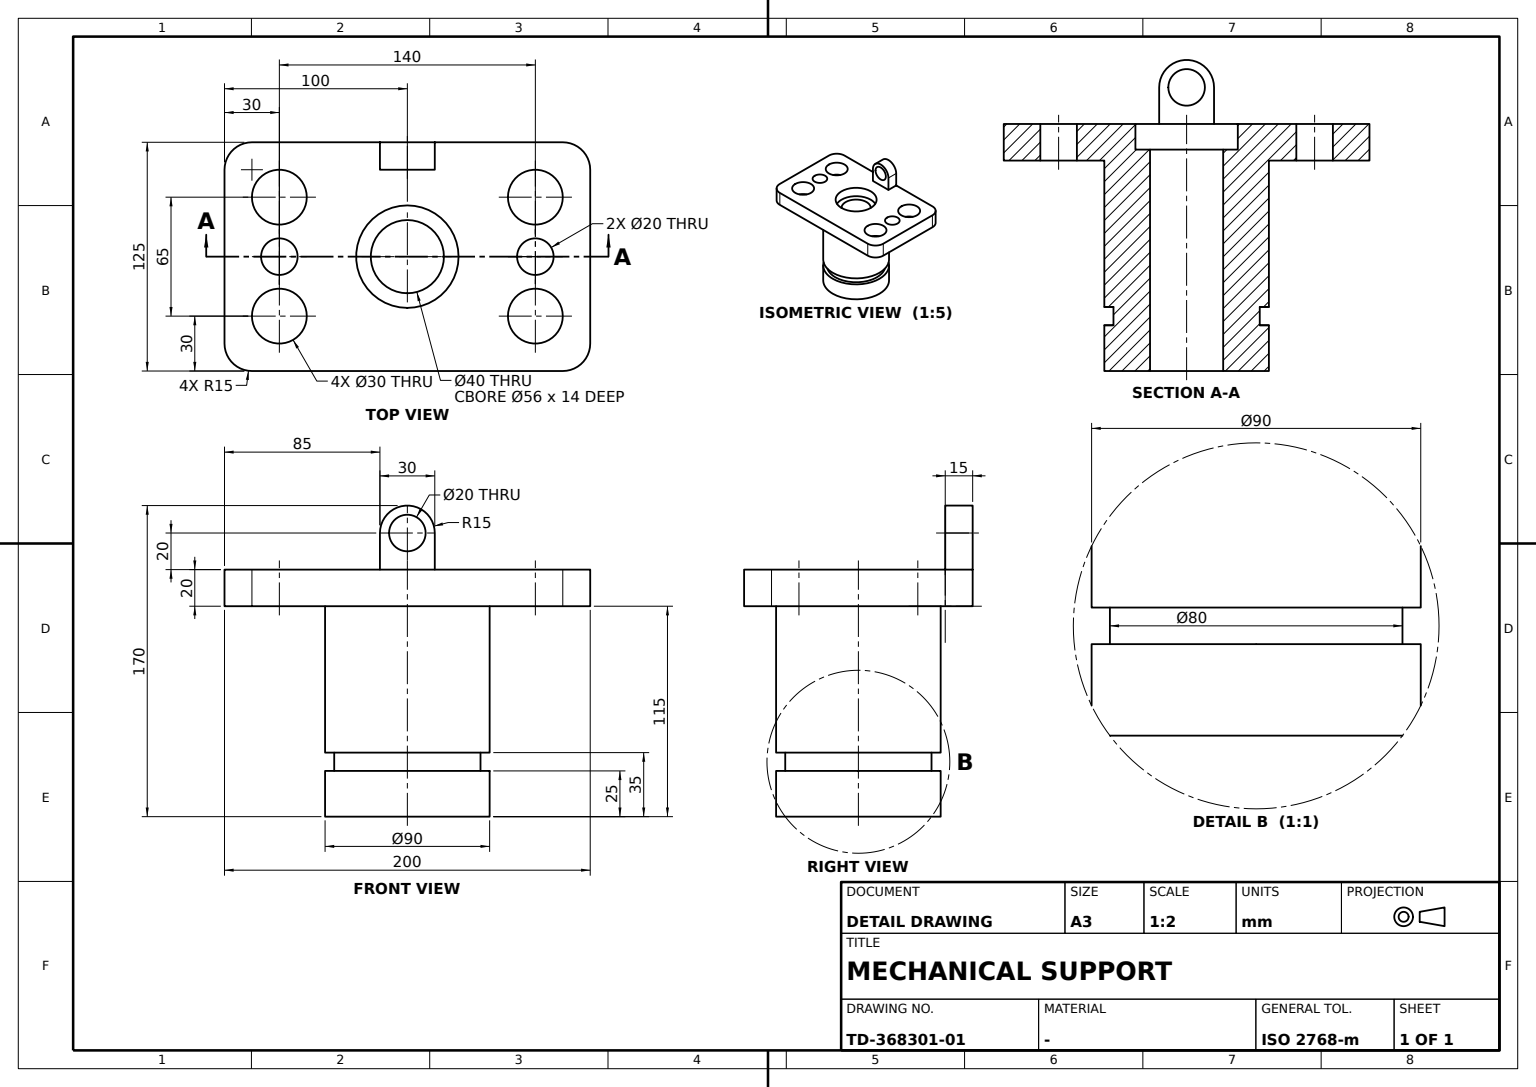
ISO-10303-21;
HEADER;
FILE_DESCRIPTION((''),'2;1');
FILE_NAME('','',(''),(''),'','','');
FILE_SCHEMA(('AUTOMOTIVE_DESIGN'));
ENDSEC;
DATA;
#1=APPLICATION_CONTEXT('');
#2=PRODUCT_CONTEXT('',#1,'mechanical');
#3=PRODUCT('','','',(#2));
#4=PRODUCT_DEFINITION_FORMATION('','',#3);
#5=PRODUCT_DEFINITION_CONTEXT('',#1,'design');
#6=PRODUCT_DEFINITION('','',#4,#5);
#7=PRODUCT_DEFINITION_SHAPE('','',#6);
#8=(LENGTH_UNIT()NAMED_UNIT(*)SI_UNIT(.MILLI.,.METRE.));
#9=(NAMED_UNIT(*)PLANE_ANGLE_UNIT()SI_UNIT($,.RADIAN.));
#10=(NAMED_UNIT(*)SI_UNIT($,.STERADIAN.)SOLID_ANGLE_UNIT());
#11=UNCERTAINTY_MEASURE_WITH_UNIT(LENGTH_MEASURE(1.E-05),#8,'distance_accuracy_value','');
#12=(GEOMETRIC_REPRESENTATION_CONTEXT(3)GLOBAL_UNCERTAINTY_ASSIGNED_CONTEXT((#11))GLOBAL_UNIT_ASSIGNED_CONTEXT((#8,#9,#10))REPRESENTATION_CONTEXT('',''));
#13=CARTESIAN_POINT('',(85.,-62.5,135.));
#14=VERTEX_POINT('',#13);
#15=CARTESIAN_POINT('',(85.,-62.5,115.));
#16=VERTEX_POINT('',#15);
#17=CARTESIAN_POINT('',(85.,-62.5,125.));
#18=DIRECTION('',(0.,0.,-1.));
#19=VECTOR('',#18,1000.);
#20=LINE('',#17,#19);
#21=EDGE_CURVE('',#14,#16,#20,.T.);
#22=ORIENTED_EDGE('',*,*,#21,.F.);
#23=CARTESIAN_POINT('',(-85.,-62.5,135.));
#24=VERTEX_POINT('',#23);
#25=CARTESIAN_POINT('',(0.,-62.5,135.));
#26=DIRECTION('',(1.,0.,0.));
#27=VECTOR('',#26,1000.);
#28=LINE('',#25,#27);
#29=EDGE_CURVE('',#24,#14,#28,.T.);
#30=ORIENTED_EDGE('',*,*,#29,.F.);
#31=CARTESIAN_POINT('',(-85.,-62.5,115.));
#32=VERTEX_POINT('',#31);
#33=CARTESIAN_POINT('',(-85.,-62.5,125.));
#34=LINE('',#33,#19);
#35=EDGE_CURVE('',#24,#32,#34,.T.);
#36=ORIENTED_EDGE('',*,*,#35,.T.);
#37=CARTESIAN_POINT('',(0.,-62.5,115.));
#38=LINE('',#37,#27);
#39=EDGE_CURVE('',#32,#16,#38,.T.);
#40=ORIENTED_EDGE('',*,*,#39,.T.);
#41=EDGE_LOOP('',(#22,#30,#36,#40));
#42=FACE_OUTER_BOUND('',#41,.T.);
#43=DIRECTION('',(0.,-1.,0.));
#44=DIRECTION('',(-1.,0.,0.));
#45=AXIS2_PLACEMENT_3D('',#13,#43,#44);
#46=PLANE('',#45);
#47=ADVANCED_FACE('',(#42),#46,.T.);
#48=CARTESIAN_POINT('',(55.,32.5,135.));
#49=VERTEX_POINT('',#48);
#50=CARTESIAN_POINT('',(85.,32.5,135.));
#51=VERTEX_POINT('',#50);
#52=CARTESIAN_POINT('',(70.,32.5,135.));
#53=DIRECTION('',(0.,0.,1.));
#54=AXIS2_PLACEMENT_3D('',#52,#53,#26);
#55=CIRCLE('',#54,15.);
#56=EDGE_CURVE('',#49,#51,#55,.T.);
#57=ORIENTED_EDGE('',*,*,#56,.F.);
#58=EDGE_CURVE('',#51,#49,#55,.T.);
#59=ORIENTED_EDGE('',*,*,#58,.F.);
#60=EDGE_LOOP('',(#57,#59));
#61=FACE_BOUND('',#60,.T.);
#62=CARTESIAN_POINT('',(0.,28.,135.));
#63=VERTEX_POINT('',#62);
#64=CARTESIAN_POINT('',(0.,-28.,135.));
#65=VERTEX_POINT('',#64);
#66=CARTESIAN_POINT('',(0.,0.,135.));
#67=AXIS2_PLACEMENT_3D('',#66,#53,#26);
#68=CIRCLE('',#67,28.);
#69=EDGE_CURVE('',#63,#65,#68,.T.);
#70=ORIENTED_EDGE('',*,*,#69,.F.);
#71=CARTESIAN_POINT('',(28.,0.,135.));
#72=VERTEX_POINT('',#71);
#73=EDGE_CURVE('',#72,#63,#68,.T.);
#74=ORIENTED_EDGE('',*,*,#73,.F.);
#75=EDGE_CURVE('',#65,#72,#68,.T.);
#76=ORIENTED_EDGE('',*,*,#75,.F.);
#77=EDGE_LOOP('',(#70,#74,#76));
#78=FACE_BOUND('',#77,.T.);
#79=CARTESIAN_POINT('',(-85.,-32.5,135.));
#80=VERTEX_POINT('',#79);
#81=CARTESIAN_POINT('',(-55.,-32.5,135.));
#82=VERTEX_POINT('',#81);
#83=CARTESIAN_POINT('',(-70.,-32.5,135.));
#84=AXIS2_PLACEMENT_3D('',#83,#53,#26);
#85=CIRCLE('',#84,15.);
#86=EDGE_CURVE('',#80,#82,#85,.T.);
#87=ORIENTED_EDGE('',*,*,#86,.F.);
#88=EDGE_CURVE('',#82,#80,#85,.T.);
#89=ORIENTED_EDGE('',*,*,#88,.F.);
#90=EDGE_LOOP('',(#87,#89));
#91=FACE_BOUND('',#90,.T.);
#92=CARTESIAN_POINT('',(-55.,32.5,135.));
#93=VERTEX_POINT('',#92);
#94=CARTESIAN_POINT('',(-85.,32.5,135.));
#95=VERTEX_POINT('',#94);
#96=CARTESIAN_POINT('',(-70.,32.5,135.));
#97=AXIS2_PLACEMENT_3D('',#96,#53,#26);
#98=CIRCLE('',#97,15.);
#99=EDGE_CURVE('',#93,#95,#98,.T.);
#100=ORIENTED_EDGE('',*,*,#99,.F.);
#101=EDGE_CURVE('',#95,#93,#98,.T.);
#102=ORIENTED_EDGE('',*,*,#101,.F.);
#103=EDGE_LOOP('',(#100,#102));
#104=FACE_BOUND('',#103,.T.);
#105=CARTESIAN_POINT('',(-80.,0.,135.));
#106=VERTEX_POINT('',#105);
#107=CARTESIAN_POINT('',(-60.,0.,135.));
#108=VERTEX_POINT('',#107);
#109=CARTESIAN_POINT('',(-70.,0.,135.));
#110=AXIS2_PLACEMENT_3D('',#109,#53,#26);
#111=CIRCLE('',#110,10.);
#112=EDGE_CURVE('',#106,#108,#111,.T.);
#113=ORIENTED_EDGE('',*,*,#112,.F.);
#114=EDGE_CURVE('',#108,#106,#111,.T.);
#115=ORIENTED_EDGE('',*,*,#114,.F.);
#116=EDGE_LOOP('',(#113,#115));
#117=FACE_BOUND('',#116,.T.);
#118=CARTESIAN_POINT('',(55.,-32.5,135.));
#119=VERTEX_POINT('',#118);
#120=CARTESIAN_POINT('',(85.,-32.5,135.));
#121=VERTEX_POINT('',#120);
#122=CARTESIAN_POINT('',(70.,-32.5,135.));
#123=AXIS2_PLACEMENT_3D('',#122,#53,#26);
#124=CIRCLE('',#123,15.);
#125=EDGE_CURVE('',#119,#121,#124,.T.);
#126=ORIENTED_EDGE('',*,*,#125,.F.);
#127=EDGE_CURVE('',#121,#119,#124,.T.);
#128=ORIENTED_EDGE('',*,*,#127,.F.);
#129=EDGE_LOOP('',(#126,#128));
#130=FACE_BOUND('',#129,.T.);
#131=CARTESIAN_POINT('',(80.,0.,135.));
#132=VERTEX_POINT('',#131);
#133=CARTESIAN_POINT('',(60.,0.,135.));
#134=VERTEX_POINT('',#133);
#135=CARTESIAN_POINT('',(70.,0.,135.));
#136=AXIS2_PLACEMENT_3D('',#135,#53,#26);
#137=CIRCLE('',#136,10.);
#138=EDGE_CURVE('',#132,#134,#137,.T.);
#139=ORIENTED_EDGE('',*,*,#138,.F.);
#140=EDGE_CURVE('',#134,#132,#137,.T.);
#141=ORIENTED_EDGE('',*,*,#140,.F.);
#142=EDGE_LOOP('',(#139,#141));
#143=FACE_BOUND('',#142,.T.);
#144=CARTESIAN_POINT('',(-100.,-47.5,135.));
#145=VERTEX_POINT('',#144);
#146=CARTESIAN_POINT('',(-85.,-47.5,135.));
#147=AXIS2_PLACEMENT_3D('',#146,#53,#26);
#148=CIRCLE('',#147,15.);
#149=EDGE_CURVE('',#145,#24,#148,.T.);
#150=ORIENTED_EDGE('',*,*,#149,.T.);
#151=ORIENTED_EDGE('',*,*,#29,.T.);
#152=CARTESIAN_POINT('',(100.,-47.5,135.));
#153=VERTEX_POINT('',#152);
#154=CARTESIAN_POINT('',(85.,-47.5,135.));
#155=AXIS2_PLACEMENT_3D('',#154,#53,#26);
#156=CIRCLE('',#155,15.);
#157=EDGE_CURVE('',#14,#153,#156,.T.);
#158=ORIENTED_EDGE('',*,*,#157,.T.);
#159=CARTESIAN_POINT('',(100.,47.5,135.));
#160=VERTEX_POINT('',#159);
#161=CARTESIAN_POINT('',(100.,0.,135.));
#162=DIRECTION('',(0.,1.,0.));
#163=VECTOR('',#162,1000.);
#164=LINE('',#161,#163);
#165=EDGE_CURVE('',#153,#160,#164,.T.);
#166=ORIENTED_EDGE('',*,*,#165,.T.);
#167=CARTESIAN_POINT('',(85.,62.5,135.));
#168=VERTEX_POINT('',#167);
#169=CARTESIAN_POINT('',(85.,47.5,135.));
#170=AXIS2_PLACEMENT_3D('',#169,#53,#26);
#171=CIRCLE('',#170,15.);
#172=EDGE_CURVE('',#160,#168,#171,.T.);
#173=ORIENTED_EDGE('',*,*,#172,.T.);
#174=CARTESIAN_POINT('',(15.,62.5,135.));
#175=VERTEX_POINT('',#174);
#176=CARTESIAN_POINT('',(50.,62.5,135.));
#177=VECTOR('',#44,1000.);
#178=LINE('',#176,#177);
#179=EDGE_CURVE('',#168,#175,#178,.T.);
#180=ORIENTED_EDGE('',*,*,#179,.T.);
#181=CARTESIAN_POINT('',(15.,47.5,135.));
#182=VERTEX_POINT('',#181);
#183=CARTESIAN_POINT('',(15.,55.,135.));
#184=VECTOR('',#43,1000.);
#185=LINE('',#183,#184);
#186=EDGE_CURVE('',#175,#182,#185,.T.);
#187=ORIENTED_EDGE('',*,*,#186,.T.);
#188=CARTESIAN_POINT('',(-15.,47.5,135.));
#189=VERTEX_POINT('',#188);
#190=CARTESIAN_POINT('',(0.,47.5,135.));
#191=LINE('',#190,#177);
#192=EDGE_CURVE('',#182,#189,#191,.T.);
#193=ORIENTED_EDGE('',*,*,#192,.T.);
#194=CARTESIAN_POINT('',(-15.,62.5,135.));
#195=VERTEX_POINT('',#194);
#196=CARTESIAN_POINT('',(-15.,55.,135.));
#197=LINE('',#196,#184);
#198=EDGE_CURVE('',#195,#189,#197,.T.);
#199=ORIENTED_EDGE('',*,*,#198,.F.);
#200=CARTESIAN_POINT('',(-85.,62.5,135.));
#201=VERTEX_POINT('',#200);
#202=CARTESIAN_POINT('',(-50.,62.5,135.));
#203=LINE('',#202,#177);
#204=EDGE_CURVE('',#195,#201,#203,.T.);
#205=ORIENTED_EDGE('',*,*,#204,.T.);
#206=CARTESIAN_POINT('',(-100.,47.5,135.));
#207=VERTEX_POINT('',#206);
#208=CARTESIAN_POINT('',(-85.,47.5,135.));
#209=AXIS2_PLACEMENT_3D('',#208,#53,#26);
#210=CIRCLE('',#209,15.);
#211=EDGE_CURVE('',#201,#207,#210,.T.);
#212=ORIENTED_EDGE('',*,*,#211,.T.);
#213=CARTESIAN_POINT('',(-100.,0.,135.));
#214=LINE('',#213,#184);
#215=EDGE_CURVE('',#207,#145,#214,.T.);
#216=ORIENTED_EDGE('',*,*,#215,.T.);
#217=EDGE_LOOP('',(#150,#151,#158,#166,#173,#180,#187,#193,#199,#205,#212,#216));
#218=FACE_OUTER_BOUND('',#217,.T.);
#219=AXIS2_PLACEMENT_3D('',#62,#53,#26);
#220=PLANE('',#219);
#221=ADVANCED_FACE('',(#61,#78,#91,#104,#117,#130,#143,#218),#220,.T.);
#222=CARTESIAN_POINT('',(0.,-40.,25.));
#223=VERTEX_POINT('',#222);
#224=CARTESIAN_POINT('',(40.,0.,25.));
#225=VERTEX_POINT('',#224);
#226=CARTESIAN_POINT('',(0.,0.,25.));
#227=AXIS2_PLACEMENT_3D('',#226,#53,#26);
#228=CIRCLE('',#227,40.);
#229=EDGE_CURVE('',#223,#225,#228,.T.);
#230=ORIENTED_EDGE('',*,*,#229,.F.);
#231=CARTESIAN_POINT('',(0.,40.,25.));
#232=VERTEX_POINT('',#231);
#233=EDGE_CURVE('',#232,#223,#228,.T.);
#234=ORIENTED_EDGE('',*,*,#233,.F.);
#235=EDGE_CURVE('',#225,#232,#228,.T.);
#236=ORIENTED_EDGE('',*,*,#235,.F.);
#237=EDGE_LOOP('',(#230,#234,#236));
#238=FACE_BOUND('',#237,.T.);
#239=CARTESIAN_POINT('',(0.,-45.,25.));
#240=VERTEX_POINT('',#239);
#241=CARTESIAN_POINT('',(45.,0.,25.));
#242=VERTEX_POINT('',#241);
#243=CIRCLE('',#227,45.);
#244=EDGE_CURVE('',#240,#242,#243,.T.);
#245=ORIENTED_EDGE('',*,*,#244,.T.);
#246=CARTESIAN_POINT('',(0.,45.,25.));
#247=VERTEX_POINT('',#246);
#248=EDGE_CURVE('',#242,#247,#243,.T.);
#249=ORIENTED_EDGE('',*,*,#248,.T.);
#250=EDGE_CURVE('',#247,#240,#243,.T.);
#251=ORIENTED_EDGE('',*,*,#250,.T.);
#252=EDGE_LOOP('',(#245,#249,#251));
#253=FACE_OUTER_BOUND('',#252,.T.);
#254=AXIS2_PLACEMENT_3D('',#231,#53,#26);
#255=PLANE('',#254);
#256=ADVANCED_FACE('',(#238,#253),#255,.T.);
#257=CARTESIAN_POINT('',(-85.,62.5,115.));
#258=VERTEX_POINT('',#257);
#259=CARTESIAN_POINT('',(-100.,47.5,115.));
#260=VERTEX_POINT('',#259);
#261=CARTESIAN_POINT('',(-85.,47.5,115.));
#262=AXIS2_PLACEMENT_3D('',#261,#53,#26);
#263=CIRCLE('',#262,15.);
#264=EDGE_CURVE('',#258,#260,#263,.T.);
#265=ORIENTED_EDGE('',*,*,#264,.T.);
#266=CARTESIAN_POINT('',(-100.,47.5,125.));
#267=LINE('',#266,#19);
#268=EDGE_CURVE('',#207,#260,#267,.T.);
#269=ORIENTED_EDGE('',*,*,#268,.F.);
#270=ORIENTED_EDGE('',*,*,#211,.F.);
#271=CARTESIAN_POINT('',(-85.,62.5,125.));
#272=LINE('',#271,#19);
#273=EDGE_CURVE('',#201,#258,#272,.T.);
#274=ORIENTED_EDGE('',*,*,#273,.T.);
#275=EDGE_LOOP('',(#265,#269,#270,#274));
#276=FACE_OUTER_BOUND('',#275,.T.);
#277=CARTESIAN_POINT('',(-85.,47.5,125.));
#278=AXIS2_PLACEMENT_3D('',#277,#18,#26);
#279=CYLINDRICAL_SURFACE('',#278,15.);
#280=ADVANCED_FACE('',(#276),#279,.T.);
#281=CARTESIAN_POINT('',(45.,0.,115.));
#282=VERTEX_POINT('',#281);
#283=CARTESIAN_POINT('',(0.,45.,115.));
#284=VERTEX_POINT('',#283);
#285=CARTESIAN_POINT('',(0.,0.,115.));
#286=AXIS2_PLACEMENT_3D('',#285,#53,#26);
#287=CIRCLE('',#286,45.);
#288=EDGE_CURVE('',#282,#284,#287,.T.);
#289=ORIENTED_EDGE('',*,*,#288,.F.);
#290=CARTESIAN_POINT('',(45.,0.,35.));
#291=VERTEX_POINT('',#290);
#292=CARTESIAN_POINT('',(45.,0.,67.5));
#293=LINE('',#292,#19);
#294=EDGE_CURVE('',#282,#291,#293,.T.);
#295=ORIENTED_EDGE('',*,*,#294,.T.);
#296=CARTESIAN_POINT('',(0.,45.,35.));
#297=VERTEX_POINT('',#296);
#298=CARTESIAN_POINT('',(0.,0.,35.));
#299=AXIS2_PLACEMENT_3D('',#298,#53,#26);
#300=CIRCLE('',#299,45.);
#301=EDGE_CURVE('',#291,#297,#300,.T.);
#302=ORIENTED_EDGE('',*,*,#301,.T.);
#303=CARTESIAN_POINT('',(0.,45.,67.5));
#304=VECTOR('',#53,1000.);
#305=LINE('',#303,#304);
#306=EDGE_CURVE('',#297,#284,#305,.T.);
#307=ORIENTED_EDGE('',*,*,#306,.T.);
#308=EDGE_LOOP('',(#289,#295,#302,#307));
#309=FACE_OUTER_BOUND('',#308,.T.);
#310=CARTESIAN_POINT('',(0.,0.,67.5));
#311=AXIS2_PLACEMENT_3D('',#310,#18,#26);
#312=CYLINDRICAL_SURFACE('',#311,45.);
#313=ADVANCED_FACE('',(#309),#312,.T.);
#314=CARTESIAN_POINT('',(80.,0.,115.));
#315=VERTEX_POINT('',#314);
#316=CARTESIAN_POINT('',(60.,0.,115.));
#317=VERTEX_POINT('',#316);
#318=CARTESIAN_POINT('',(70.,0.,115.));
#319=AXIS2_PLACEMENT_3D('',#318,#53,#26);
#320=CIRCLE('',#319,10.);
#321=EDGE_CURVE('',#315,#317,#320,.T.);
#322=ORIENTED_EDGE('',*,*,#321,.F.);
#323=CARTESIAN_POINT('',(80.,0.,125.));
#324=LINE('',#323,#19);
#325=EDGE_CURVE('',#132,#315,#324,.T.);
#326=ORIENTED_EDGE('',*,*,#325,.F.);
#327=ORIENTED_EDGE('',*,*,#138,.T.);
#328=CARTESIAN_POINT('',(60.,0.,125.));
#329=LINE('',#328,#19);
#330=EDGE_CURVE('',#134,#317,#329,.T.);
#331=ORIENTED_EDGE('',*,*,#330,.T.);
#332=EDGE_LOOP('',(#322,#326,#327,#331));
#333=FACE_OUTER_BOUND('',#332,.T.);
#334=CARTESIAN_POINT('',(70.,0.,125.));
#335=AXIS2_PLACEMENT_3D('',#334,#18,#26);
#336=CYLINDRICAL_SURFACE('',#335,10.);
#337=ADVANCED_FACE('',(#333),#336,.F.);
#338=CARTESIAN_POINT('',(85.,-32.5,115.));
#339=VERTEX_POINT('',#338);
#340=CARTESIAN_POINT('',(85.,-32.5,125.));
#341=LINE('',#340,#19);
#342=EDGE_CURVE('',#121,#339,#341,.T.);
#343=ORIENTED_EDGE('',*,*,#342,.T.);
#344=CARTESIAN_POINT('',(55.,-32.5,115.));
#345=VERTEX_POINT('',#344);
#346=CARTESIAN_POINT('',(70.,-32.5,115.));
#347=AXIS2_PLACEMENT_3D('',#346,#53,#26);
#348=CIRCLE('',#347,15.);
#349=EDGE_CURVE('',#345,#339,#348,.T.);
#350=ORIENTED_EDGE('',*,*,#349,.F.);
#351=CARTESIAN_POINT('',(55.,-32.5,125.));
#352=LINE('',#351,#19);
#353=EDGE_CURVE('',#119,#345,#352,.T.);
#354=ORIENTED_EDGE('',*,*,#353,.F.);
#355=ORIENTED_EDGE('',*,*,#125,.T.);
#356=EDGE_LOOP('',(#343,#350,#354,#355));
#357=FACE_OUTER_BOUND('',#356,.T.);
#358=CARTESIAN_POINT('',(70.,-32.5,125.));
#359=AXIS2_PLACEMENT_3D('',#358,#18,#26);
#360=CYLINDRICAL_SURFACE('',#359,15.);
#361=ADVANCED_FACE('',(#357),#360,.F.);
#362=CARTESIAN_POINT('',(40.,0.,35.));
#363=VERTEX_POINT('',#362);
#364=CARTESIAN_POINT('',(40.,0.,67.5));
#365=LINE('',#364,#19);
#366=EDGE_CURVE('',#363,#225,#365,.T.);
#367=ORIENTED_EDGE('',*,*,#366,.F.);
#368=CARTESIAN_POINT('',(0.,-40.,35.));
#369=VERTEX_POINT('',#368);
#370=CIRCLE('',#299,40.);
#371=EDGE_CURVE('',#369,#363,#370,.T.);
#372=ORIENTED_EDGE('',*,*,#371,.F.);
#373=CARTESIAN_POINT('',(0.,-40.,30.));
#374=LINE('',#373,#304);
#375=EDGE_CURVE('',#223,#369,#374,.T.);
#376=ORIENTED_EDGE('',*,*,#375,.F.);
#377=ORIENTED_EDGE('',*,*,#229,.T.);
#378=EDGE_LOOP('',(#367,#372,#376,#377));
#379=FACE_OUTER_BOUND('',#378,.T.);
#380=CYLINDRICAL_SURFACE('',#311,40.);
#381=ADVANCED_FACE('',(#379),#380,.T.);
#382=CARTESIAN_POINT('',(-10.,47.5,155.));
#383=VERTEX_POINT('',#382);
#384=CARTESIAN_POINT('',(10.,47.5,155.));
#385=VERTEX_POINT('',#384);
#386=CARTESIAN_POINT('',(0.,47.5,155.));
#387=AXIS2_PLACEMENT_3D('',#386,#162,#44);
#388=CIRCLE('',#387,10.);
#389=EDGE_CURVE('',#383,#385,#388,.T.);
#390=ORIENTED_EDGE('',*,*,#389,.T.);
#391=EDGE_CURVE('',#385,#383,#388,.T.);
#392=ORIENTED_EDGE('',*,*,#391,.T.);
#393=EDGE_LOOP('',(#390,#392));
#394=FACE_BOUND('',#393,.T.);
#395=CARTESIAN_POINT('',(15.,47.5,155.));
#396=VERTEX_POINT('',#395);
#397=CARTESIAN_POINT('',(15.,47.5,145.));
#398=LINE('',#397,#19);
#399=EDGE_CURVE('',#396,#182,#398,.T.);
#400=ORIENTED_EDGE('',*,*,#399,.F.);
#401=CARTESIAN_POINT('',(-15.,47.5,155.));
#402=VERTEX_POINT('',#401);
#403=CIRCLE('',#387,15.);
#404=EDGE_CURVE('',#402,#396,#403,.T.);
#405=ORIENTED_EDGE('',*,*,#404,.F.);
#406=CARTESIAN_POINT('',(-15.,47.5,145.));
#407=LINE('',#406,#304);
#408=EDGE_CURVE('',#189,#402,#407,.T.);
#409=ORIENTED_EDGE('',*,*,#408,.F.);
#410=ORIENTED_EDGE('',*,*,#192,.F.);
#411=EDGE_LOOP('',(#400,#405,#409,#410));
#412=FACE_OUTER_BOUND('',#411,.T.);
#413=CARTESIAN_POINT('',(0.,47.5,0.));
#414=AXIS2_PLACEMENT_3D('',#413,#162,#44);
#415=PLANE('',#414);
#416=ADVANCED_FACE('',(#394,#412),#415,.F.);
#417=ORIENTED_EDGE('',*,*,#21,.T.);
#418=CARTESIAN_POINT('',(100.,-47.5,115.));
#419=VERTEX_POINT('',#418);
#420=CARTESIAN_POINT('',(85.,-47.5,115.));
#421=AXIS2_PLACEMENT_3D('',#420,#53,#26);
#422=CIRCLE('',#421,15.);
#423=EDGE_CURVE('',#16,#419,#422,.T.);
#424=ORIENTED_EDGE('',*,*,#423,.T.);
#425=CARTESIAN_POINT('',(100.,-47.5,125.));
#426=LINE('',#425,#19);
#427=EDGE_CURVE('',#153,#419,#426,.T.);
#428=ORIENTED_EDGE('',*,*,#427,.F.);
#429=ORIENTED_EDGE('',*,*,#157,.F.);
#430=EDGE_LOOP('',(#417,#424,#428,#429));
#431=FACE_OUTER_BOUND('',#430,.T.);
#432=CARTESIAN_POINT('',(85.,-47.5,125.));
#433=AXIS2_PLACEMENT_3D('',#432,#18,#26);
#434=CYLINDRICAL_SURFACE('',#433,15.);
#435=ADVANCED_FACE('',(#431),#434,.T.);
#436=ORIENTED_EDGE('',*,*,#114,.T.);
#437=CARTESIAN_POINT('',(-80.,0.,115.));
#438=VERTEX_POINT('',#437);
#439=CARTESIAN_POINT('',(-80.,0.,125.));
#440=LINE('',#439,#19);
#441=EDGE_CURVE('',#106,#438,#440,.T.);
#442=ORIENTED_EDGE('',*,*,#441,.T.);
#443=CARTESIAN_POINT('',(-60.,0.,115.));
#444=VERTEX_POINT('',#443);
#445=CARTESIAN_POINT('',(-70.,0.,115.));
#446=AXIS2_PLACEMENT_3D('',#445,#53,#26);
#447=CIRCLE('',#446,10.);
#448=EDGE_CURVE('',#444,#438,#447,.T.);
#449=ORIENTED_EDGE('',*,*,#448,.F.);
#450=CARTESIAN_POINT('',(-60.,0.,125.));
#451=LINE('',#450,#19);
#452=EDGE_CURVE('',#108,#444,#451,.T.);
#453=ORIENTED_EDGE('',*,*,#452,.F.);
#454=EDGE_LOOP('',(#436,#442,#449,#453));
#455=FACE_OUTER_BOUND('',#454,.T.);
#456=CARTESIAN_POINT('',(-70.,0.,125.));
#457=AXIS2_PLACEMENT_3D('',#456,#18,#26);
#458=CYLINDRICAL_SURFACE('',#457,10.);
#459=ADVANCED_FACE('',(#455),#458,.F.);
#460=ORIENTED_EDGE('',*,*,#56,.T.);
#461=CARTESIAN_POINT('',(85.,32.5,115.));
#462=VERTEX_POINT('',#461);
#463=CARTESIAN_POINT('',(85.,32.5,125.));
#464=LINE('',#463,#19);
#465=EDGE_CURVE('',#51,#462,#464,.T.);
#466=ORIENTED_EDGE('',*,*,#465,.T.);
#467=CARTESIAN_POINT('',(55.,32.5,115.));
#468=VERTEX_POINT('',#467);
#469=CARTESIAN_POINT('',(70.,32.5,115.));
#470=AXIS2_PLACEMENT_3D('',#469,#53,#26);
#471=CIRCLE('',#470,15.);
#472=EDGE_CURVE('',#468,#462,#471,.T.);
#473=ORIENTED_EDGE('',*,*,#472,.F.);
#474=CARTESIAN_POINT('',(55.,32.5,125.));
#475=LINE('',#474,#19);
#476=EDGE_CURVE('',#49,#468,#475,.T.);
#477=ORIENTED_EDGE('',*,*,#476,.F.);
#478=EDGE_LOOP('',(#460,#466,#473,#477));
#479=FACE_OUTER_BOUND('',#478,.T.);
#480=CARTESIAN_POINT('',(70.,32.5,125.));
#481=AXIS2_PLACEMENT_3D('',#480,#18,#26);
#482=CYLINDRICAL_SURFACE('',#481,15.);
#483=ADVANCED_FACE('',(#479),#482,.F.);
#484=ORIENTED_EDGE('',*,*,#404,.T.);
#485=CARTESIAN_POINT('',(15.,62.5,155.));
#486=VERTEX_POINT('',#485);
#487=CARTESIAN_POINT('',(15.,55.,155.));
#488=LINE('',#487,#184);
#489=EDGE_CURVE('',#486,#396,#488,.T.);
#490=ORIENTED_EDGE('',*,*,#489,.F.);
#491=CARTESIAN_POINT('',(-15.,62.5,155.));
#492=VERTEX_POINT('',#491);
#493=CARTESIAN_POINT('',(0.,62.5,155.));
#494=AXIS2_PLACEMENT_3D('',#493,#162,#44);
#495=CIRCLE('',#494,15.);
#496=EDGE_CURVE('',#492,#486,#495,.T.);
#497=ORIENTED_EDGE('',*,*,#496,.F.);
#498=CARTESIAN_POINT('',(-15.,55.,155.));
#499=LINE('',#498,#184);
#500=EDGE_CURVE('',#492,#402,#499,.T.);
#501=ORIENTED_EDGE('',*,*,#500,.T.);
#502=EDGE_LOOP('',(#484,#490,#497,#501));
#503=FACE_OUTER_BOUND('',#502,.T.);
#504=CARTESIAN_POINT('',(0.,55.,155.));
#505=AXIS2_PLACEMENT_3D('',#504,#43,#44);
#506=CYLINDRICAL_SURFACE('',#505,15.);
#507=ADVANCED_FACE('',(#503),#506,.T.);
#508=CARTESIAN_POINT('',(0.,20.,121.));
#509=VERTEX_POINT('',#508);
#510=CARTESIAN_POINT('',(0.,20.,0.));
#511=VERTEX_POINT('',#510);
#512=CARTESIAN_POINT('',(0.,20.,60.5));
#513=LINE('',#512,#19);
#514=EDGE_CURVE('',#509,#511,#513,.T.);
#515=ORIENTED_EDGE('',*,*,#514,.T.);
#516=CARTESIAN_POINT('',(20.,0.,0.));
#517=VERTEX_POINT('',#516);
#518=CARTESIAN_POINT('',(0.,0.,0.));
#519=AXIS2_PLACEMENT_3D('',#518,#53,#26);
#520=CIRCLE('',#519,20.);
#521=EDGE_CURVE('',#517,#511,#520,.T.);
#522=ORIENTED_EDGE('',*,*,#521,.F.);
#523=CARTESIAN_POINT('',(20.,0.,121.));
#524=VERTEX_POINT('',#523);
#525=CARTESIAN_POINT('',(20.,0.,67.5));
#526=LINE('',#525,#19);
#527=EDGE_CURVE('',#524,#517,#526,.T.);
#528=ORIENTED_EDGE('',*,*,#527,.F.);
#529=CARTESIAN_POINT('',(0.,0.,121.));
#530=AXIS2_PLACEMENT_3D('',#529,#53,#26);
#531=CIRCLE('',#530,20.);
#532=EDGE_CURVE('',#524,#509,#531,.T.);
#533=ORIENTED_EDGE('',*,*,#532,.T.);
#534=EDGE_LOOP('',(#515,#522,#528,#533));
#535=FACE_OUTER_BOUND('',#534,.T.);
#536=CYLINDRICAL_SURFACE('',#311,20.);
#537=ADVANCED_FACE('',(#535),#536,.F.);
#538=ORIENTED_EDGE('',*,*,#325,.T.);
#539=EDGE_CURVE('',#317,#315,#320,.T.);
#540=ORIENTED_EDGE('',*,*,#539,.F.);
#541=ORIENTED_EDGE('',*,*,#330,.F.);
#542=ORIENTED_EDGE('',*,*,#140,.T.);
#543=EDGE_LOOP('',(#538,#540,#541,#542));
#544=FACE_OUTER_BOUND('',#543,.T.);
#545=ADVANCED_FACE('',(#544),#336,.F.);
#546=CARTESIAN_POINT('',(85.,62.5,115.));
#547=VERTEX_POINT('',#546);
#548=CARTESIAN_POINT('',(85.,62.5,125.));
#549=LINE('',#548,#19);
#550=EDGE_CURVE('',#168,#547,#549,.T.);
#551=ORIENTED_EDGE('',*,*,#550,.F.);
#552=ORIENTED_EDGE('',*,*,#172,.F.);
#553=CARTESIAN_POINT('',(100.,47.5,115.));
#554=VERTEX_POINT('',#553);
#555=CARTESIAN_POINT('',(100.,47.5,125.));
#556=LINE('',#555,#19);
#557=EDGE_CURVE('',#160,#554,#556,.T.);
#558=ORIENTED_EDGE('',*,*,#557,.T.);
#559=CARTESIAN_POINT('',(85.,47.5,115.));
#560=AXIS2_PLACEMENT_3D('',#559,#53,#26);
#561=CIRCLE('',#560,15.);
#562=EDGE_CURVE('',#554,#547,#561,.T.);
#563=ORIENTED_EDGE('',*,*,#562,.T.);
#564=EDGE_LOOP('',(#551,#552,#558,#563));
#565=FACE_OUTER_BOUND('',#564,.T.);
#566=CARTESIAN_POINT('',(85.,47.5,125.));
#567=AXIS2_PLACEMENT_3D('',#566,#18,#26);
#568=CYLINDRICAL_SURFACE('',#567,15.);
#569=ADVANCED_FACE('',(#565),#568,.T.);
#570=ORIENTED_EDGE('',*,*,#375,.T.);
#571=CARTESIAN_POINT('',(0.,40.,35.));
#572=VERTEX_POINT('',#571);
#573=EDGE_CURVE('',#572,#369,#370,.T.);
#574=ORIENTED_EDGE('',*,*,#573,.F.);
#575=CARTESIAN_POINT('',(0.,40.,30.));
#576=LINE('',#575,#304);
#577=EDGE_CURVE('',#232,#572,#576,.T.);
#578=ORIENTED_EDGE('',*,*,#577,.F.);
#579=ORIENTED_EDGE('',*,*,#233,.T.);
#580=EDGE_LOOP('',(#570,#574,#578,#579));
#581=FACE_OUTER_BOUND('',#580,.T.);
#582=ADVANCED_FACE('',(#581),#380,.T.);
#583=CARTESIAN_POINT('',(28.,0.,121.));
#584=VERTEX_POINT('',#583);
#585=CARTESIAN_POINT('',(0.,28.,121.));
#586=VERTEX_POINT('',#585);
#587=CIRCLE('',#530,28.);
#588=EDGE_CURVE('',#584,#586,#587,.T.);
#589=ORIENTED_EDGE('',*,*,#588,.F.);
#590=CARTESIAN_POINT('',(28.,0.,67.5));
#591=LINE('',#590,#19);
#592=EDGE_CURVE('',#72,#584,#591,.T.);
#593=ORIENTED_EDGE('',*,*,#592,.F.);
#594=ORIENTED_EDGE('',*,*,#73,.T.);
#595=CARTESIAN_POINT('',(0.,28.,128.));
#596=LINE('',#595,#19);
#597=EDGE_CURVE('',#63,#586,#596,.T.);
#598=ORIENTED_EDGE('',*,*,#597,.T.);
#599=EDGE_LOOP('',(#589,#593,#594,#598));
#600=FACE_OUTER_BOUND('',#599,.T.);
#601=CYLINDRICAL_SURFACE('',#311,28.);
#602=ADVANCED_FACE('',(#600),#601,.F.);
#603=ORIENTED_EDGE('',*,*,#288,.T.);
#604=CARTESIAN_POINT('',(0.,-45.,115.));
#605=VERTEX_POINT('',#604);
#606=EDGE_CURVE('',#284,#605,#287,.T.);
#607=ORIENTED_EDGE('',*,*,#606,.T.);
#608=EDGE_CURVE('',#605,#282,#287,.T.);
#609=ORIENTED_EDGE('',*,*,#608,.T.);
#610=EDGE_LOOP('',(#603,#607,#609));
#611=FACE_BOUND('',#610,.T.);
#612=CARTESIAN_POINT('',(-85.,-32.5,115.));
#613=VERTEX_POINT('',#612);
#614=CARTESIAN_POINT('',(-55.,-32.5,115.));
#615=VERTEX_POINT('',#614);
#616=CARTESIAN_POINT('',(-70.,-32.5,115.));
#617=AXIS2_PLACEMENT_3D('',#616,#53,#26);
#618=CIRCLE('',#617,15.);
#619=EDGE_CURVE('',#613,#615,#618,.T.);
#620=ORIENTED_EDGE('',*,*,#619,.T.);
#621=EDGE_CURVE('',#615,#613,#618,.T.);
#622=ORIENTED_EDGE('',*,*,#621,.T.);
#623=EDGE_LOOP('',(#620,#622));
#624=FACE_BOUND('',#623,.T.);
#625=EDGE_CURVE('',#462,#468,#471,.T.);
#626=ORIENTED_EDGE('',*,*,#625,.T.);
#627=ORIENTED_EDGE('',*,*,#472,.T.);
#628=EDGE_LOOP('',(#626,#627));
#629=FACE_BOUND('',#628,.T.);
#630=EDGE_CURVE('',#339,#345,#348,.T.);
#631=ORIENTED_EDGE('',*,*,#630,.T.);
#632=ORIENTED_EDGE('',*,*,#349,.T.);
#633=EDGE_LOOP('',(#631,#632));
#634=FACE_BOUND('',#633,.T.);
#635=CARTESIAN_POINT('',(0.,62.5,115.));
#636=LINE('',#635,#177);
#637=EDGE_CURVE('',#547,#258,#636,.T.);
#638=ORIENTED_EDGE('',*,*,#637,.F.);
#639=ORIENTED_EDGE('',*,*,#562,.F.);
#640=CARTESIAN_POINT('',(100.,0.,115.));
#641=LINE('',#640,#163);
#642=EDGE_CURVE('',#419,#554,#641,.T.);
#643=ORIENTED_EDGE('',*,*,#642,.F.);
#644=ORIENTED_EDGE('',*,*,#423,.F.);
#645=ORIENTED_EDGE('',*,*,#39,.F.);
#646=CARTESIAN_POINT('',(-100.,-47.5,115.));
#647=VERTEX_POINT('',#646);
#648=CARTESIAN_POINT('',(-85.,-47.5,115.));
#649=AXIS2_PLACEMENT_3D('',#648,#53,#26);
#650=CIRCLE('',#649,15.);
#651=EDGE_CURVE('',#647,#32,#650,.T.);
#652=ORIENTED_EDGE('',*,*,#651,.F.);
#653=CARTESIAN_POINT('',(-100.,0.,115.));
#654=LINE('',#653,#184);
#655=EDGE_CURVE('',#260,#647,#654,.T.);
#656=ORIENTED_EDGE('',*,*,#655,.F.);
#657=ORIENTED_EDGE('',*,*,#264,.F.);
#658=EDGE_LOOP('',(#638,#639,#643,#644,#645,#652,#656,#657));
#659=FACE_OUTER_BOUND('',#658,.T.);
#660=ORIENTED_EDGE('',*,*,#321,.T.);
#661=ORIENTED_EDGE('',*,*,#539,.T.);
#662=EDGE_LOOP('',(#660,#661));
#663=FACE_BOUND('',#662,.T.);
#664=ORIENTED_EDGE('',*,*,#448,.T.);
#665=EDGE_CURVE('',#438,#444,#447,.T.);
#666=ORIENTED_EDGE('',*,*,#665,.T.);
#667=EDGE_LOOP('',(#664,#666));
#668=FACE_BOUND('',#667,.T.);
#669=CARTESIAN_POINT('',(-55.,32.5,115.));
#670=VERTEX_POINT('',#669);
#671=CARTESIAN_POINT('',(-85.,32.5,115.));
#672=VERTEX_POINT('',#671);
#673=CARTESIAN_POINT('',(-70.,32.5,115.));
#674=AXIS2_PLACEMENT_3D('',#673,#53,#26);
#675=CIRCLE('',#674,15.);
#676=EDGE_CURVE('',#670,#672,#675,.T.);
#677=ORIENTED_EDGE('',*,*,#676,.T.);
#678=EDGE_CURVE('',#672,#670,#675,.T.);
#679=ORIENTED_EDGE('',*,*,#678,.T.);
#680=EDGE_LOOP('',(#677,#679));
#681=FACE_BOUND('',#680,.T.);
#682=PLANE('',#286);
#683=ADVANCED_FACE('',(#611,#624,#629,#634,#659,#663,#668,#681),#682,.F.);
#684=ORIENTED_EDGE('',*,*,#101,.T.);
#685=CARTESIAN_POINT('',(-55.,32.5,125.));
#686=LINE('',#685,#19);
#687=EDGE_CURVE('',#93,#670,#686,.T.);
#688=ORIENTED_EDGE('',*,*,#687,.T.);
#689=ORIENTED_EDGE('',*,*,#678,.F.);
#690=CARTESIAN_POINT('',(-85.,32.5,125.));
#691=LINE('',#690,#19);
#692=EDGE_CURVE('',#95,#672,#691,.T.);
#693=ORIENTED_EDGE('',*,*,#692,.F.);
#694=EDGE_LOOP('',(#684,#688,#689,#693));
#695=FACE_OUTER_BOUND('',#694,.T.);
#696=CARTESIAN_POINT('',(-70.,32.5,125.));
#697=AXIS2_PLACEMENT_3D('',#696,#18,#26);
#698=CYLINDRICAL_SURFACE('',#697,15.);
#699=ADVANCED_FACE('',(#695),#698,.F.);
#700=ORIENTED_EDGE('',*,*,#389,.F.);
#701=CARTESIAN_POINT('',(-10.,62.5,155.));
#702=VERTEX_POINT('',#701);
#703=CARTESIAN_POINT('',(-10.,55.,155.));
#704=LINE('',#703,#184);
#705=EDGE_CURVE('',#702,#383,#704,.T.);
#706=ORIENTED_EDGE('',*,*,#705,.F.);
#707=CARTESIAN_POINT('',(10.,62.5,155.));
#708=VERTEX_POINT('',#707);
#709=CIRCLE('',#494,10.);
#710=EDGE_CURVE('',#702,#708,#709,.T.);
#711=ORIENTED_EDGE('',*,*,#710,.T.);
#712=CARTESIAN_POINT('',(10.,55.,155.));
#713=LINE('',#712,#184);
#714=EDGE_CURVE('',#708,#385,#713,.T.);
#715=ORIENTED_EDGE('',*,*,#714,.T.);
#716=EDGE_LOOP('',(#700,#706,#711,#715));
#717=FACE_OUTER_BOUND('',#716,.T.);
#718=CYLINDRICAL_SURFACE('',#505,10.);
#719=ADVANCED_FACE('',(#717),#718,.F.);
#720=CARTESIAN_POINT('',(0.,-45.,35.));
#721=VERTEX_POINT('',#720);
#722=CARTESIAN_POINT('',(0.,-45.,67.5));
#723=LINE('',#722,#304);
#724=EDGE_CURVE('',#721,#605,#723,.T.);
#725=ORIENTED_EDGE('',*,*,#724,.F.);
#726=EDGE_CURVE('',#721,#291,#300,.T.);
#727=ORIENTED_EDGE('',*,*,#726,.T.);
#728=ORIENTED_EDGE('',*,*,#294,.F.);
#729=ORIENTED_EDGE('',*,*,#608,.F.);
#730=EDGE_LOOP('',(#725,#727,#728,#729));
#731=FACE_OUTER_BOUND('',#730,.T.);
#732=ADVANCED_FACE('',(#731),#312,.T.);
#733=ORIENTED_EDGE('',*,*,#86,.T.);
#734=CARTESIAN_POINT('',(-55.,-32.5,125.));
#735=LINE('',#734,#19);
#736=EDGE_CURVE('',#82,#615,#735,.T.);
#737=ORIENTED_EDGE('',*,*,#736,.T.);
#738=ORIENTED_EDGE('',*,*,#619,.F.);
#739=CARTESIAN_POINT('',(-85.,-32.5,125.));
#740=LINE('',#739,#19);
#741=EDGE_CURVE('',#80,#613,#740,.T.);
#742=ORIENTED_EDGE('',*,*,#741,.F.);
#743=EDGE_LOOP('',(#733,#737,#738,#742));
#744=FACE_OUTER_BOUND('',#743,.T.);
#745=CARTESIAN_POINT('',(-70.,-32.5,125.));
#746=AXIS2_PLACEMENT_3D('',#745,#18,#26);
#747=CYLINDRICAL_SURFACE('',#746,15.);
#748=ADVANCED_FACE('',(#744),#747,.F.);
#749=CARTESIAN_POINT('',(0.,-45.,0.));
#750=VERTEX_POINT('',#749);
#751=EDGE_CURVE('',#750,#240,#723,.T.);
#752=ORIENTED_EDGE('',*,*,#751,.F.);
#753=CARTESIAN_POINT('',(45.,0.,0.));
#754=VERTEX_POINT('',#753);
#755=CIRCLE('',#519,45.);
#756=EDGE_CURVE('',#750,#754,#755,.T.);
#757=ORIENTED_EDGE('',*,*,#756,.T.);
#758=EDGE_CURVE('',#242,#754,#293,.T.);
#759=ORIENTED_EDGE('',*,*,#758,.F.);
#760=ORIENTED_EDGE('',*,*,#244,.F.);
#761=EDGE_LOOP('',(#752,#757,#759,#760));
#762=FACE_OUTER_BOUND('',#761,.T.);
#763=ADVANCED_FACE('',(#762),#312,.T.);
#764=ORIENTED_EDGE('',*,*,#248,.F.);
#765=ORIENTED_EDGE('',*,*,#758,.T.);
#766=CARTESIAN_POINT('',(0.,45.,0.));
#767=VERTEX_POINT('',#766);
#768=EDGE_CURVE('',#754,#767,#755,.T.);
#769=ORIENTED_EDGE('',*,*,#768,.T.);
#770=EDGE_CURVE('',#767,#247,#305,.T.);
#771=ORIENTED_EDGE('',*,*,#770,.T.);
#772=EDGE_LOOP('',(#764,#765,#769,#771));
#773=FACE_OUTER_BOUND('',#772,.T.);
#774=ADVANCED_FACE('',(#773),#312,.T.);
#775=EDGE_CURVE('',#297,#721,#300,.T.);
#776=ORIENTED_EDGE('',*,*,#775,.T.);
#777=ORIENTED_EDGE('',*,*,#724,.T.);
#778=ORIENTED_EDGE('',*,*,#606,.F.);
#779=ORIENTED_EDGE('',*,*,#306,.F.);
#780=EDGE_LOOP('',(#776,#777,#778,#779));
#781=FACE_OUTER_BOUND('',#780,.T.);
#782=ADVANCED_FACE('',(#781),#312,.T.);
#783=ORIENTED_EDGE('',*,*,#705,.T.);
#784=ORIENTED_EDGE('',*,*,#391,.F.);
#785=ORIENTED_EDGE('',*,*,#714,.F.);
#786=EDGE_CURVE('',#708,#702,#709,.T.);
#787=ORIENTED_EDGE('',*,*,#786,.T.);
#788=EDGE_LOOP('',(#783,#784,#785,#787));
#789=FACE_OUTER_BOUND('',#788,.T.);
#790=ADVANCED_FACE('',(#789),#718,.F.);
#791=ORIENTED_EDGE('',*,*,#399,.T.);
#792=ORIENTED_EDGE('',*,*,#186,.F.);
#793=CARTESIAN_POINT('',(15.,62.5,145.));
#794=LINE('',#793,#19);
#795=EDGE_CURVE('',#486,#175,#794,.T.);
#796=ORIENTED_EDGE('',*,*,#795,.F.);
#797=ORIENTED_EDGE('',*,*,#489,.T.);
#798=EDGE_LOOP('',(#791,#792,#796,#797));
#799=FACE_OUTER_BOUND('',#798,.T.);
#800=AXIS2_PLACEMENT_3D('',#174,#26,#53);
#801=PLANE('',#800);
#802=ADVANCED_FACE('',(#799),#801,.T.);
#803=ORIENTED_EDGE('',*,*,#366,.T.);
#804=ORIENTED_EDGE('',*,*,#235,.T.);
#805=ORIENTED_EDGE('',*,*,#577,.T.);
#806=EDGE_CURVE('',#363,#572,#370,.T.);
#807=ORIENTED_EDGE('',*,*,#806,.F.);
#808=EDGE_LOOP('',(#803,#804,#805,#807));
#809=FACE_OUTER_BOUND('',#808,.T.);
#810=ADVANCED_FACE('',(#809),#380,.T.);
#811=ORIENTED_EDGE('',*,*,#655,.T.);
#812=CARTESIAN_POINT('',(-100.,-47.5,125.));
#813=LINE('',#812,#19);
#814=EDGE_CURVE('',#145,#647,#813,.T.);
#815=ORIENTED_EDGE('',*,*,#814,.F.);
#816=ORIENTED_EDGE('',*,*,#215,.F.);
#817=ORIENTED_EDGE('',*,*,#268,.T.);
#818=EDGE_LOOP('',(#811,#815,#816,#817));
#819=FACE_OUTER_BOUND('',#818,.T.);
#820=AXIS2_PLACEMENT_3D('',#144,#44,#162);
#821=PLANE('',#820);
#822=ADVANCED_FACE('',(#819),#821,.T.);
#823=ORIENTED_EDGE('',*,*,#665,.F.);
#824=ORIENTED_EDGE('',*,*,#441,.F.);
#825=ORIENTED_EDGE('',*,*,#112,.T.);
#826=ORIENTED_EDGE('',*,*,#452,.T.);
#827=EDGE_LOOP('',(#823,#824,#825,#826));
#828=FACE_OUTER_BOUND('',#827,.T.);
#829=ADVANCED_FACE('',(#828),#458,.F.);
#830=ORIENTED_EDGE('',*,*,#768,.F.);
#831=ORIENTED_EDGE('',*,*,#756,.F.);
#832=EDGE_CURVE('',#767,#750,#755,.T.);
#833=ORIENTED_EDGE('',*,*,#832,.F.);
#834=EDGE_LOOP('',(#830,#831,#833));
#835=FACE_OUTER_BOUND('',#834,.T.);
#836=ORIENTED_EDGE('',*,*,#521,.T.);
#837=CARTESIAN_POINT('',(0.,-20.,0.));
#838=VERTEX_POINT('',#837);
#839=EDGE_CURVE('',#511,#838,#520,.T.);
#840=ORIENTED_EDGE('',*,*,#839,.T.);
#841=EDGE_CURVE('',#838,#517,#520,.T.);
#842=ORIENTED_EDGE('',*,*,#841,.T.);
#843=EDGE_LOOP('',(#836,#840,#842));
#844=FACE_BOUND('',#843,.T.);
#845=AXIS2_PLACEMENT_3D('',#766,#53,#26);
#846=PLANE('',#845);
#847=ADVANCED_FACE('',(#835,#844),#846,.F.);
#848=ORIENTED_EDGE('',*,*,#35,.F.);
#849=ORIENTED_EDGE('',*,*,#149,.F.);
#850=ORIENTED_EDGE('',*,*,#814,.T.);
#851=ORIENTED_EDGE('',*,*,#651,.T.);
#852=EDGE_LOOP('',(#848,#849,#850,#851));
#853=FACE_OUTER_BOUND('',#852,.T.);
#854=CARTESIAN_POINT('',(-85.,-47.5,125.));
#855=AXIS2_PLACEMENT_3D('',#854,#18,#26);
#856=CYLINDRICAL_SURFACE('',#855,15.);
#857=ADVANCED_FACE('',(#853),#856,.T.);
#858=ORIENTED_EDGE('',*,*,#751,.T.);
#859=ORIENTED_EDGE('',*,*,#250,.F.);
#860=ORIENTED_EDGE('',*,*,#770,.F.);
#861=ORIENTED_EDGE('',*,*,#832,.T.);
#862=EDGE_LOOP('',(#858,#859,#860,#861));
#863=FACE_OUTER_BOUND('',#862,.T.);
#864=ADVANCED_FACE('',(#863),#312,.T.);
#865=ORIENTED_EDGE('',*,*,#527,.T.);
#866=ORIENTED_EDGE('',*,*,#841,.F.);
#867=CARTESIAN_POINT('',(0.,-20.,121.));
#868=VERTEX_POINT('',#867);
#869=CARTESIAN_POINT('',(0.,-20.,60.5));
#870=LINE('',#869,#19);
#871=EDGE_CURVE('',#868,#838,#870,.T.);
#872=ORIENTED_EDGE('',*,*,#871,.F.);
#873=EDGE_CURVE('',#868,#524,#531,.T.);
#874=ORIENTED_EDGE('',*,*,#873,.T.);
#875=EDGE_LOOP('',(#865,#866,#872,#874));
#876=FACE_OUTER_BOUND('',#875,.T.);
#877=ADVANCED_FACE('',(#876),#536,.F.);
#878=ORIENTED_EDGE('',*,*,#99,.T.);
#879=ORIENTED_EDGE('',*,*,#692,.T.);
#880=ORIENTED_EDGE('',*,*,#676,.F.);
#881=ORIENTED_EDGE('',*,*,#687,.F.);
#882=EDGE_LOOP('',(#878,#879,#880,#881));
#883=FACE_OUTER_BOUND('',#882,.T.);
#884=ADVANCED_FACE('',(#883),#698,.F.);
#885=ORIENTED_EDGE('',*,*,#642,.T.);
#886=ORIENTED_EDGE('',*,*,#557,.F.);
#887=ORIENTED_EDGE('',*,*,#165,.F.);
#888=ORIENTED_EDGE('',*,*,#427,.T.);
#889=EDGE_LOOP('',(#885,#886,#887,#888));
#890=FACE_OUTER_BOUND('',#889,.T.);
#891=AXIS2_PLACEMENT_3D('',#159,#26,#43);
#892=PLANE('',#891);
#893=ADVANCED_FACE('',(#890),#892,.T.);
#894=ORIENTED_EDGE('',*,*,#514,.F.);
#895=EDGE_CURVE('',#509,#868,#531,.T.);
#896=ORIENTED_EDGE('',*,*,#895,.T.);
#897=ORIENTED_EDGE('',*,*,#871,.T.);
#898=ORIENTED_EDGE('',*,*,#839,.F.);
#899=EDGE_LOOP('',(#894,#896,#897,#898));
#900=FACE_OUTER_BOUND('',#899,.T.);
#901=ADVANCED_FACE('',(#900),#536,.F.);
#902=ORIENTED_EDGE('',*,*,#630,.F.);
#903=ORIENTED_EDGE('',*,*,#342,.F.);
#904=ORIENTED_EDGE('',*,*,#127,.T.);
#905=ORIENTED_EDGE('',*,*,#353,.T.);
#906=EDGE_LOOP('',(#902,#903,#904,#905));
#907=FACE_OUTER_BOUND('',#906,.T.);
#908=ADVANCED_FACE('',(#907),#360,.F.);
#909=CARTESIAN_POINT('',(0.,-28.,121.));
#910=VERTEX_POINT('',#909);
#911=EDGE_CURVE('',#586,#910,#587,.T.);
#912=ORIENTED_EDGE('',*,*,#911,.T.);
#913=EDGE_CURVE('',#910,#584,#587,.T.);
#914=ORIENTED_EDGE('',*,*,#913,.T.);
#915=ORIENTED_EDGE('',*,*,#588,.T.);
#916=EDGE_LOOP('',(#912,#914,#915));
#917=FACE_OUTER_BOUND('',#916,.T.);
#918=ORIENTED_EDGE('',*,*,#873,.F.);
#919=ORIENTED_EDGE('',*,*,#895,.F.);
#920=ORIENTED_EDGE('',*,*,#532,.F.);
#921=EDGE_LOOP('',(#918,#919,#920));
#922=FACE_BOUND('',#921,.T.);
#923=AXIS2_PLACEMENT_3D('',#508,#53,#26);
#924=PLANE('',#923);
#925=ADVANCED_FACE('',(#917,#922),#924,.T.);
#926=ORIENTED_EDGE('',*,*,#913,.F.);
#927=CARTESIAN_POINT('',(0.,-28.,128.));
#928=LINE('',#927,#19);
#929=EDGE_CURVE('',#65,#910,#928,.T.);
#930=ORIENTED_EDGE('',*,*,#929,.F.);
#931=ORIENTED_EDGE('',*,*,#75,.T.);
#932=ORIENTED_EDGE('',*,*,#592,.T.);
#933=EDGE_LOOP('',(#926,#930,#931,#932));
#934=FACE_OUTER_BOUND('',#933,.T.);
#935=ADVANCED_FACE('',(#934),#601,.F.);
#936=CARTESIAN_POINT('',(-15.,62.5,145.));
#937=LINE('',#936,#304);
#938=EDGE_CURVE('',#195,#492,#937,.T.);
#939=ORIENTED_EDGE('',*,*,#938,.F.);
#940=ORIENTED_EDGE('',*,*,#198,.T.);
#941=ORIENTED_EDGE('',*,*,#408,.T.);
#942=ORIENTED_EDGE('',*,*,#500,.F.);
#943=EDGE_LOOP('',(#939,#940,#941,#942));
#944=FACE_OUTER_BOUND('',#943,.T.);
#945=AXIS2_PLACEMENT_3D('',#194,#26,#53);
#946=PLANE('',#945);
#947=ADVANCED_FACE('',(#944),#946,.F.);
#948=ORIENTED_EDGE('',*,*,#929,.T.);
#949=ORIENTED_EDGE('',*,*,#911,.F.);
#950=ORIENTED_EDGE('',*,*,#597,.F.);
#951=ORIENTED_EDGE('',*,*,#69,.T.);
#952=EDGE_LOOP('',(#948,#949,#950,#951));
#953=FACE_OUTER_BOUND('',#952,.T.);
#954=ADVANCED_FACE('',(#953),#601,.F.);
#955=ORIENTED_EDGE('',*,*,#736,.F.);
#956=ORIENTED_EDGE('',*,*,#88,.T.);
#957=ORIENTED_EDGE('',*,*,#741,.T.);
#958=ORIENTED_EDGE('',*,*,#621,.F.);
#959=EDGE_LOOP('',(#955,#956,#957,#958));
#960=FACE_OUTER_BOUND('',#959,.T.);
#961=ADVANCED_FACE('',(#960),#747,.F.);
#962=ORIENTED_EDGE('',*,*,#710,.F.);
#963=ORIENTED_EDGE('',*,*,#786,.F.);
#964=EDGE_LOOP('',(#962,#963));
#965=FACE_BOUND('',#964,.T.);
#966=ORIENTED_EDGE('',*,*,#938,.T.);
#967=ORIENTED_EDGE('',*,*,#496,.T.);
#968=ORIENTED_EDGE('',*,*,#795,.T.);
#969=ORIENTED_EDGE('',*,*,#179,.F.);
#970=ORIENTED_EDGE('',*,*,#550,.T.);
#971=ORIENTED_EDGE('',*,*,#637,.T.);
#972=ORIENTED_EDGE('',*,*,#273,.F.);
#973=ORIENTED_EDGE('',*,*,#204,.F.);
#974=EDGE_LOOP('',(#966,#967,#968,#969,#970,#971,#972,#973));
#975=FACE_OUTER_BOUND('',#974,.T.);
#976=AXIS2_PLACEMENT_3D('',#200,#162,#26);
#977=PLANE('',#976);
#978=ADVANCED_FACE('',(#965,#975),#977,.T.);
#979=ORIENTED_EDGE('',*,*,#58,.T.);
#980=ORIENTED_EDGE('',*,*,#476,.T.);
#981=ORIENTED_EDGE('',*,*,#625,.F.);
#982=ORIENTED_EDGE('',*,*,#465,.F.);
#983=EDGE_LOOP('',(#979,#980,#981,#982));
#984=FACE_OUTER_BOUND('',#983,.T.);
#985=ADVANCED_FACE('',(#984),#482,.F.);
#986=ORIENTED_EDGE('',*,*,#573,.T.);
#987=ORIENTED_EDGE('',*,*,#371,.T.);
#988=ORIENTED_EDGE('',*,*,#806,.T.);
#989=EDGE_LOOP('',(#986,#987,#988));
#990=FACE_BOUND('',#989,.T.);
#991=ORIENTED_EDGE('',*,*,#726,.F.);
#992=ORIENTED_EDGE('',*,*,#775,.F.);
#993=ORIENTED_EDGE('',*,*,#301,.F.);
#994=EDGE_LOOP('',(#991,#992,#993));
#995=FACE_OUTER_BOUND('',#994,.T.);
#996=AXIS2_PLACEMENT_3D('',#296,#53,#26);
#997=PLANE('',#996);
#998=ADVANCED_FACE('',(#990,#995),#997,.F.);
#999=CLOSED_SHELL('',(#47,#221,#256,#280,#313,#337,#361,#381,#416,#435,#459,#483,#507,#537,#545,#569,#582,#602,#683,#699,#719,#732,#748,#763,#774,#782,#790,#802,#810,#822,#829,#847,#857,#864,#877,#884,#893,#901,#908,#925,#935,#947,#954,#961,#978,#985,#998));
#1000=MANIFOLD_SOLID_BREP('',#999);
#1001=ADVANCED_BREP_SHAPE_REPRESENTATION('',(#1000),#12);
#1002=SHAPE_DEFINITION_REPRESENTATION(#7,#1001);
ENDSEC;
END-ISO-10303-21;
